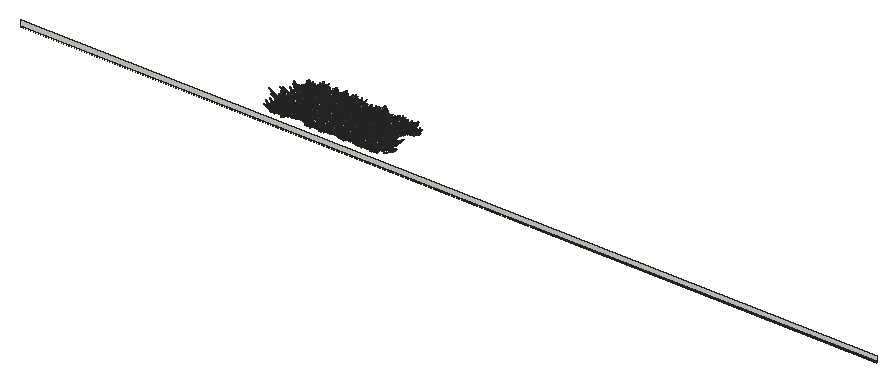
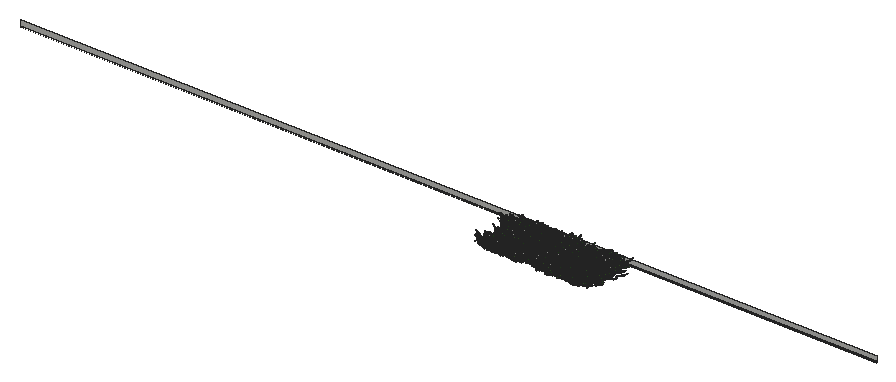
# SketchUp Ruby script. Lengths in inches.
U = 1.inch
M = Sketchup.active_model
def pt(a) = Geom::Point3d.new(a.map { |v| v * U })
def face(e, loops, mat)
  f = e.add_face(loops[0].map { |a| pt(a) })
  loops[1..].each { |l| e.add_face(l.map { |a| pt(a) }).erase! }
  f.material = f.back_material = mat if mat
  f
end
# faces: each face lists its corners as indices into pts; further lists are holes
def faces(e, pts, list, mat = nil) = list.each { |f| face(e, (f[0].is_a?(Array) ? f : [f]).map { |l| l.map { |i| pts[i] } }, mat) }
# xy, xz, yz: faces in a plane at the given z, y or x. An outline is a flat list of corners, or four numbers for a rectangle; further outlines are holes
def ring(l) = l.size == 4 ? [[l[0], l[1]], [l[2], l[1]], [l[2], l[3]], [l[0], l[3]]] : l.each_slice(2).to_a
def flat(e, list, mat, &to3) = list.each { |f| face(e, (f[0].is_a?(Array) ? f : [f]).map { |l| ring(l).map { |u, v| to3.(u, v) } }, mat) }
def xy(e, z, list, mat = nil) = flat(e, list, mat) { |x, y| [x, y, z] }
def xz(e, y, list, mat = nil) = flat(e, list, mat) { |x, z| [x, y, z] }
def yz(e, x, list, mat = nil) = flat(e, list, mat) { |y, z| [x, y, z] }
def lines(e, pts, list) = list.each { |a, b| e.add_line(pt(pts[a]), pt(pts[b])) }
# prism: a flat outline (further loops are holes) pulled along v
def prism(e, loops, v, mat = nil)
  f = face(e, loops, mat); d = Geom::Vector3d.new(v.map { |x| x * U })
  f.pushpull(f.normal.samedirection?(d) ? d.length : -d.length)
end
def box(e, o, s, mat = nil) = prism(e, [[o, [o[0] + s[0], o[1], o[2]], [o[0] + s[0], o[1] + s[1], o[2]], [o[0], o[1] + s[1], o[2]]]], [0, 0, s[2]], mat)
def at(x, y, z, deg = 0) = Geom::Transformation.translation(pt([x, y, z])) * Geom::Transformation.rotation(ORIGIN, Z_AXIS, deg.degrees)
def axes(o, x, y, z) = Geom::Transformation.new([*x, 0, *y, 0, *z, 0, *pt(o).to_a, 1])
def part(name) = M.definitions.add(name)
# library, detail: a bought-in or finely detailed component or shape, given as its bounding box
def library(name, o, s) = part(name).tap { |d| box(d.entities, o, s) }
def detail(e, o, s) = box(e.add_group.entities, o, s)
def put(e, d, t, mat = nil) = e.add_instance(d, t).tap { |i| i.material = mat if mat }
def group(e, t, mat = nil) = e.add_group.tap { |g| g.transformation = t; g.material = mat if mat }.entities
root = M.entities
M.materials.add("Material82").color = [68, 110, 58]
M.materials.add("Material83").color = [48, 90, 38]
M.materials.add("Material84").color = [68, 110, 48]
M.materials.add("Material85").color = [48, 90, 48]
M.materials.add("Material86").color = [58, 110, 58]
M.materials.add("Material87").color = [58, 90, 38]
M.materials.add("Material88").color = [68, 100, 58]
M.materials.add("Material89").color = [48, 100, 38]
c1 = part("grass00")
p = [[-0.6875,0.15,0],[-0.56,0.08,5.52],[-0.04,0.03,2.76],[0.48,-0.02,0],[0.35,-0.02,5.52],[-0.1,-0.14,5.52],
  [-0.12,0.65,8.37],[-0.42,0.65,8.37]]
faces(c1.entities,p,[[0,1,2,3],[3,2,4],[1,5,2],[5,4,2],[1,6,5],[4,5,6],[7,6,1]])
c2 = part("Group16\#1")
put(c2.entities,c1,axes([1.44,-0.61,-0.01],[0.05352,0.12609,0],[-0.10704,0.04543,0.07239],[0.06664,-0.02828,0.11628]),"Material85")
put(c2.entities,c1,axes([0.76,-0.15,-0.01],[0.04676,0.24062,0],[-0.23162,0.04501,0.06642],[0.0652,-0.01267,0.23595]),"Material82")
put(c2.entities,c1,axes([0.79,0.01,-0.01],[-0.00606,0.34651,0],[-0.34381,-0.00602,0.0432],[0.04319,0.00076,0.34386]))
put(c2.entities,c1,axes([1,0.23,-0.01],[-0.07192,0.31144,0],[-0.28722,-0.06632,0.1236],[0.12043,0.02781,0.29478]),"Material84")
put(c2.entities,c1,axes([1.66,0.77,-0.01],[-0.13828,0.29651,0],[-0.21551,-0.1005,0.22471],[0.20365,0.09498,0.23779]),"Material89")
put(c2.entities,c1,axes([0.6875,0.52,-0.01],[-0.18126,0.24051,0],[-0.22746,-0.17142,0.09788],[0.07817,0.05891,0.28481]),"Material84")
put(c2.entities,c1,axes([0.68,0.78,-0.01],[-0.215,0.18688,0],[-0.12385,-0.14248,0.21334],[0.13995,0.16101,0.18878]),"Material82")
put(c2.entities,c1,axes([0.56,1,-0.01],[-0.13756,0.07624,0],[-0.06159,-0.11112,0.0927],[0.04494,0.08108,0.12705]),"Material84")
put(c2.entities,c1,axes([0.2,0.64,-0.01],[-0.23729,0.07254,0],[-0.05711,-0.18681,0.153],[0.04473,0.14632,0.19535]),"Material89")
put(c2.entities,c1,axes([0.0625,0.72,-0.01],[-0.28874,0.02525,0],[-0.02179,-0.24916,0.14647],[0.01276,0.14591,0.25012]),"Material82")
put(c2.entities,c1,axes([-0.08,0.62,-0.01],[-0.34089,-0.04187,0],[0.03255,-0.26504,0.216],[-0.02633,0.21439,0.26703]),"Material89")
put(c2.entities,c1,axes([-0.34,0.98,-0.01],[-0.14314,-0.0493,0],[0.04397,-0.12769,0.06843],[-0.02228,0.0647,0.13505]),"Material89")
put(c2.entities,c1,axes([-0.87,1.45,-0.01],[-0.23488,-0.14114,0],[0.13761,-0.22901,0.06087],[-0.03135,0.05217,0.26717]))
put(c2.entities,c1,axes([-0.72,0.77,-0.01],[-0.14208,-0.13251,0],[0.07209,-0.0773,0.16301],[-0.11118,0.11922,0.1057]),"Material89")
put(c2.entities,c1,axes([-0.62,0.43,-0.01],[-0.14845,-0.21203,0],[0.18654,-0.13061,0.12304],[-0.10079,0.07057,0.22772]),"Material82")
put(c2.entities,c1,axes([-0.68,0.29,-0.01],[-0.13639,-0.32136,0],[0.31723,-0.13464,0.05579],[-0.05136,0.0218,0.34462]),"Material83")
put(c2.entities,c1,axes([-0.64,0.125,-0.01],[-0.0458,-0.23569,0],[0.22124,-0.043,0.08276],[-0.08124,0.01579,0.22538]),"Material86")
put(c2.entities,c1,axes([-1.6,-0.03,-0.01],[0.00576,-0.32897,0],[0.27526,0.00482,0.18018],[-0.18015,-0.00315,0.2753]),"Material84")
put(c2.entities,c1,axes([-1.36,-0.31,-0.01],[0.05718,-0.24765,0],[0.18172,0.04196,0.17267],[-0.16825,-0.03885,0.1865]),"Material89")
put(c2.entities,c1,axes([-1.54,-0.72,-0.01],[0.06537,-0.14017,0],[0.13555,0.06321,0.03939],[-0.0357,-0.01665,0.14956]))
put(c2.entities,c1,axes([-1.19,-0.9,-0.01],[0.09597,-0.12735,0],[0.11214,0.08451,0.07557],[-0.06035,-0.04548,0.14042]),"Material88")
put(c2.entities,c1,axes([-0.47,-0.54,-0.01],[0.11588,-0.10072,0],[0.0618,0.0711,0.12124],[-0.07953,-0.0915,0.0942]))
put(c2.entities,c1,axes([-0.47,-0.84,-0.01],[0.11927,-0.0661,0],[0.06603,0.11913,0.00646],[-0.00313,-0.00565,0.13621]),"Material84")
put(c2.entities,c1,axes([-0.38,-1.24,-0.01],[0.28037,-0.08571,0],[0.0618,0.20215,0.20315],[-0.05939,-0.19428,0.21139]),"Material88")
put(c2.entities,c1,axes([-0.06,-0.66,-0.01],[0.22719,-0.01987,0],[0.01247,0.14255,0.17758],[-0.01547,-0.17691,0.1431]),"Material87")
put(c2.entities,c1,axes([0.11,-0.89,-0.01],[0.14882,0.01828,0],[-0.01058,0.08611,0.12229],[0.01491,-0.12138,0.08676]),"Material85")
put(c2.entities,c1,axes([0.25,-0.72,-0.01],[0.20481,0.07053,0],[-0.06206,0.18022,0.10291],[0.03351,-0.0973,0.1906]),"Material85")
put(c2.entities,c1,axes([0.85,-1.42,-0.01],[0.16481,0.09904,0],[-0.09472,0.15762,0.05616],[0.02893,-0.04814,0.18389]),"Material84")
put(c2.entities,c1,axes([1.01,-1.09,-0.01],[0.21858,0.20385,0],[-0.17495,0.1876,0.15339],[0.10462,-0.11218,0.25652]),"Material89")
put(c2.entities,c1,axes([1.01,-0.71,-0.01],[0.08733,0.12473,0],[-0.06445,0.04512,0.13037],[0.1068,-0.07477,0.07867]),"Material85")
c3 = part("Group15\#1")
put(c3.entities,c2,at(0,0,0))
c4 = part("3darcstudiotree_grass00\#1")
put(c4.entities,c3,at(0,0,0))
xz(root,273.41,[[1534.73,-38.1875,2096.97,-37.86],[1534.73,-37.24,2096.97,-34.17]])
put(root,c4,axes([1753.47,281.1875,-34.17],[2.17079,-1.3067,0],[3.53732,0.91396,-0.04807],[0.21538,0.05565,1.69791]))
put(root,c4,axes([1759.32,281.2,-34.17],[4.07054,-0.47424,0],[1.26442,1.68794,-0.05518],[0.08285,0.1106,1.77288]))
put(root,c4,axes([1699.04,281.26,-34.17],[0.55958,-1.81201,0],[3.80263,0.18264,-0.0324],[0.16574,0.00796,1.47946]))
put(root,c4,axes([1722.34,281.33,-34.17],[1.12764,-1.73077,0],[4.18377,0.42395,-0.01129],[0.06303,0.00639,1.86628]))
put(root,c4,axes([1743.74,281.47,-34.17],[1.22394,-1.54587,0],[4.34445,0.53497,-0.04262],[0.21661,0.02667,1.81655]))
put(root,c4,axes([1732.14,281.62,-34.17],[-3.03372,-1.40875,0],[3.08967,-1.03482,-0.05304],[0.26,-0.08708,1.95407]))
put(root,c4,axes([1727.11,282.65,-34.17],[1.40551,-1.64885,0],[4.26228,0.56508,-0.02131],[0.10181,0.0135,1.69918]))
put(root,c4,axes([1731.34,282.95,-34.17],[1.31732,-1.5277,0],[3.94533,0.52911,-0.01889],[0.1126,0.0151,1.96679]))
put(root,c4,axes([1754.46,283.05,-34.17],[1.63405,-1.64828,0],[3.24927,0.50099,-0.00888],[0.05923,0.00913,1.87213]))
put(root,c4,axes([1701,282.59,-34.17],[-3.98203,-0.87024,0],[2.1917,-1.55976,-0.02403],[0.066,-0.04697,1.92026]))
put(root,c4,axes([1748.21,282.77,-34.17],[-3.61082,-0.39433,0],[1.20081,-1.71014,-0.02644],[0.03989,-0.05681,1.9068]))
put(root,c4,axes([1710.51,282.87,-34.17],[-3.87962,-0.67736,0],[1.4284,-1.27243,-0.0129],[0.02606,-0.02321,1.31952]))
put(root,c4,axes([1745.46,283.12,-34.17],[3.46015,0.38109,0],[-0.88814,1.25417,-0.03829],[-0.05842,0.0825,1.40372]))
put(root,c4,axes([1740.78,282.8,-34.17],[-3.41936,-0.32293,0],[0.80872,-1.33182,-0.00326],[0.00565,-0.00931,1.93944]))
put(root,c4,axes([1723.11,283.16,-34.17],[3.02481,0.98705,0],[-2.84435,1.35567,-0.00662],[-0.02068,0.00986,1.63949]))
put(root,c4,axes([1718.68,283.8,-34.17],[0.88446,1.28365,0],[-3.4154,0.366,-0.02204],[-0.14997,0.01607,1.87051]))
put(root,c4,axes([1705.0625,283.9,-34.17],[-0.33098,1.70392,0],[-3.92143,-0.11847,-0.03234],[-0.20787,-0.00628,1.90052]))
put(root,c4,axes([1705.14,284.73,-34.17],[4.23456,-0.44217,0],[1.03247,1.53783,-0.03329],[0.03822,0.05692,1.35616]))
put(root,c4,axes([1753.52,284.58,-34.17],[-1.01765,1.47435,0],[-4.56253,-0.4898,-0.0223],[-0.09653,-0.01036,1.58974]))
put(root,c4,axes([1712.44,284.81,-34.17],[0.47172,1.49628,0],[-3.52699,0.17294,-0.00588],[-0.02991,0.00147,1.36568]))
put(root,c4,axes([1760.9,285.43,-34.17],[0.9992,-1.70874,0],[3.78612,0.34433,-0.00305],[0.01806,0.00164,1.76865]))
put(root,c4,axes([1735.08,285.14,-34.17],[-3.90096,-0.14279,0],[0.42836,-1.82008,-0.06502],[0.0247,-0.10495,1.42798]))
put(root,c4,axes([1749.08,285.56,-34.17],[4.57837,0.42186,0],[-0.79113,1.33536,-0.04207],[-0.04884,0.08244,1.32997]))
put(root,c4,axes([1717.02,285.52,-34.17],[1.5336,1.30723,0],[-4.13356,0.75421,-0.03574],[-0.18177,0.03317,1.91331]))
put(root,c4,axes([1722.26,286,-34.17],[3.57543,-0.38769,0],[0.94849,1.36047,-0.03828],[0.05948,0.08532,1.57185]))
put(root,c4,axes([1743.97,286.02,-34.17],[3.20776,-0.47754,0],[1.28857,1.34619,-0.04981],[0.10847,0.11332,1.68613]))
put(root,c4,axes([1726.58,285.74,-34.17],[0.98392,1.60393,0],[-4.31274,0.41147,-0.01063],[-0.04621,0.00441,1.48723]))
put(root,c4,axes([1698.96,286.05,-34.17],[-2.94402,-0.61655,0],[1.96985,-1.46292,-0.05452],[0.11404,-0.08469,1.404]))
put(root,c4,axes([1761.52,286.76,-34.17],[0.83554,-1.66698,0],[4.46376,0.34798,-0.04547],[0.22573,0.0176,1.72572]))
put(root,c4,axes([1739.54,286.08,-34.17],[-4.29885,0.51765,0],[-1.3445,-1.73657,-0.03433],[-0.03931,-0.05078,1.35329]))
put(root,c4,axes([1745.2,286.72,-34.17],[-0.83396,-1.47678,0],[3.24144,-0.28469,-0.00779],[0.04244,-0.00373,1.38852]))
put(root,c4,axes([1749.99,287,-34.17],[0.8669,-1.63737,0],[4.38165,0.36081,-0.01659],[0.07514,0.00619,1.55232]))
put(root,c4,axes([1734.67,286.9,-34.17],[2.831,1.13552,0],[-3.26481,1.26594,-0.00938],[-0.03813,0.01479,1.95578]))
put(root,c4,axes([1727.38,286.87,-34.17],[2.31946,1.24356,0],[-3.54601,1.02866,-0.02079],[-0.06877,0.01995,1.35493]))
put(root,c4,axes([1716.98,287.19,-34.17],[3.58882,-0.43849,0],[1.01017,1.28588,-0.04073],[0.06773,0.08621,1.43775]))
put(root,c4,axes([1710.05,287.42,-34.17],[3.87508,-0.19158,0],[0.55593,1.74888,-0.03701],[0.02742,0.08626,1.99511]))
put(root,c4,axes([1755.1,286.81,-34.17],[-1.66334,1.46333,0],[-4.128,-0.72978,-0.00369],[-0.01567,-0.00277,1.57624]))
put(root,c4,axes([1701.35,287.47,-34.17],[-2.23453,-0.97852,0],[2.77364,-0.9851,-0.04825],[0.23755,-0.08437,1.85346]))
put(root,c4,axes([1737.07,288.01,-34.17],[0.13943,1.51336,0],[-3.52829,0.05056,-0.04285],[-0.2957,0.00424,1.82733]))
put(root,c4,axes([1722.85,287.92,-34.17],[-2.1552,1.3099,0],[-3.57978,-0.91604,-0.05659],[-0.20761,-0.05313,1.39892]))
put(root,c4,axes([1706.03,288.18,-34.17],[-3.02099,1.21639,0],[-3.37871,-1.30508,-0.0181],[-0.07062,-0.02728,1.93624]))
put(root,c4,axes([1712.21,288.95,-34.17],[4.11072,0.52115,0],[-1.12592,1.38127,-0.00634],[-0.01225,0.01503,1.74238]))
put(root,c4,axes([1699.97,289.22,-34.17],[1.39356,-1.72752,0],[4.38256,0.54985,-0.00448],[0.02218,0.00278,1.79011]))
put(root,c4,axes([1759.64,289.61,-34.17],[-0.53843,-1.61653,0],[3.48383,-0.18047,-0.04534],[0.27707,-0.01435,1.62314]))
put(root,c4,axes([1754.86,289.17,-34.17],[-1.88196,1.3957,0],[-3.10758,-0.65171,-0.04799],[-0.32006,-0.06712,1.99284]))
put(root,c4,axes([1704.65,289.95,-34.17],[0.57397,-1.69302,0],[4.41794,0.23295,-0.0102],[0.05353,0.00282,1.76846]))
put(root,c4,axes([1738.95,289.83,-34.17],[-0.52019,-1.47295,0],[3.61124,-0.19836,-0.01078],[0.07028,-0.00386,1.79898]))
put(root,c4,axes([1742.48,289.66,-34.17],[-0.97814,1.51943,0],[-3.80237,-0.3807,-0.01715],[-0.08253,-0.00826,1.46021]))
put(root,c4,axes([1724.19,289.77,-34.17],[0.84595,1.74988,0],[-3.45616,0.25986,-0.03349],[-0.2005,0.01508,1.60736]))
put(root,c4,axes([1715.28,290,-34.17],[-3.51608,0.58555,0],[-1.76508,-1.64843,-0.01449],[-0.02729,-0.02549,1.64714]))
put(root,c4,axes([1751.16,290.39,-34.17],[2.67266,1.37649,0],[-3.28703,0.99263,-0.02004],[-0.06999,0.02114,1.3651]))
put(root,c4,axes([1725.6875,290.53,-34.17],[-2.74028,-0.81988,0],[2.08475,-1.08371,-0.01586],[0.05642,-0.02933,1.52204]))
put(root,c4,axes([1731.9375,290.22,-34.17],[-2.48253,1.23787,0],[-2.67891,-0.83558,-0.01059],[-0.04346,-0.01356,1.33934]))
put(root,c4,axes([1728.22,291.375,-34.17],[-3.00354,-1.31894,0],[3.37135,-1.19405,-0.05274],[0.22952,-0.08129,1.98669]))
put(root,c4,axes([1735.15,291.86,-34.17],[1.37504,-1.64012,0],[4.21946,0.55019,-0.04027],[0.19656,0.02563,1.71232]))
put(root,c4,axes([1751.53,292.11,-34.17],[2.76982,-1.52047,0],[2.85461,0.80878,-0.0087],[0.04308,0.01221,1.60603]))
put(root,c4,axes([1711.15,292.1875,-34.17],[2.88399,-0.92183,0],[2.75264,1.33938,-0.02341],[0.07157,0.03482,1.59067]))
put(root,c4,axes([1722.84,291.59,-34.17],[-4.47684,0.54828,0],[-1.1065,-1.40519,-0.03919],[-0.07055,-0.08959,1.69748]))
put(root,c4,axes([1753.65,291.6,-34.17],[-4.11453,0.51388,0],[-1.13165,-1.40923,-0.01419],[-0.02668,-0.03323,1.75006]))
put(root,c4,axes([1737.4,291.6875,-34.17],[-4.23608,0.30685,0],[-0.85226,-1.82987,-0.05609],[-0.05564,-0.11947,1.94158]))
put(root,c4,axes([1745.36,291.95,-34.17],[2.07706,1.01263,0],[-2.63538,0.84072,-0.02717],[-0.1514,0.0483,1.82093]))
put(root,c4,axes([1759.7,291.98,-34.17],[-3.63945,-0.58666,0],[1.30533,-1.25945,-0.04864],[0.1019,-0.09832,1.4319]))
put(root,c4,axes([1706.06,292.07,-34.17],[-4.25916,-0.67423,0],[1.26133,-1.23925,-0.04034],[0.09396,-0.09232,1.58691]))
put(root,c4,axes([1698.41,291.66,-34.17],[-3.70599,0.79197,0],[-2.20745,-1.60656,-0.0133],[-0.03552,-0.02585,1.94738]))
put(root,c4,axes([1714.98,292.51,-34.17],[-4.16919,-0.21002,0],[0.49933,-1.5417,-0.0157],[0.01299,-0.04011,1.92971]))
put(root,c4,axes([1699.76,293.28,-34.17],[-0.43315,-1.7077,0],[3.80872,-0.15025,-0.05423],[0.31945,-0.0126,1.69842]))
put(root,c4,axes([1722.02,293.84,-34.17],[1.31559,-1.26739,0],[3.71813,0.60026,-0.00546],[0.02236,0.00361,1.33158]))
put(root,c4,axes([1733.34,293.35,-34.17],[0.02685,1.39613,0],[-4.67009,0.01397,-0.03677],[-0.14547,0.00044,1.38481]))
put(root,c4,axes([1729.65,293.98,-34.17],[2.75881,-1.06303,0],[3.05708,1.23394,-0.03867],[0.14354,0.05794,1.7417]))
put(root,c4,axes([1711.7,293.77,-34.17],[-1.10259,-1.32087,0],[4.19794,-0.54501,-0.05688],[0.29749,-0.03862,1.82396]))
put(root,c4,axes([1757.14,294.25,-34.17],[0.84647,-1.73268,0],[3.98325,0.30265,-0.00212],[0.01137,0.00086,1.6588]))
put(root,c4,axes([1750.33,293.55,-34.17],[-2.78854,1.36928,0],[-2.88748,-0.91457,-0.04358],[-0.20411,-0.06465,1.66757]))
put(root,c4,axes([1737.88,294.65,-34.17],[3.75686,0.07381,0],[-0.21994,1.74119,-0.00527],[-0.00126,0.00998,1.59512]))
put(root,c4,axes([1703.72,294.69,-34.17],[2.35188,-1.38482,0],[3.12769,0.82614,-0.05113],[0.23612,0.06237,1.56833]))
put(root,c4,axes([1743.79,294.06,-34.17],[-2.45653,1.59128,0],[-3.13753,-0.75331,-0.03488],[-0.14833,-0.03561,1.37068]))
put(root,c4,axes([1715.22,294.87,-34.17],[0.70204,1.43301,0],[-3.58325,0.27302,-0.03785],[-0.19362,0.01475,1.42505]))
put(root,c4,axes([1751.76,296.27,-34.17],[3.07151,-0.57195,0],[1.60637,1.34169,-0.03456],[0.08725,0.07287,1.66747]))
put(root,c4,axes([1745.32,296.33,-34.17],[0.41064,-1.32496,0],[4.30887,0.2077,-0.02785],[0.12721,0.00613,1.49696]))
put(root,c4,axes([1715.5625,296.54,-34.17],[3.86131,0.54377,0],[-1.4335,1.58316,-0.00059],[-0.00108,0.0012,1.74794]))
put(root,c4,axes([1712.33,296.25,-34.17],[-3.05685,-0.82947,0],[2.14696,-1.23058,-0.02104],[0.07287,-0.04177,1.73448]))
put(root,c4,axes([1726.47,296.72,-34.17],[2.41246,-1.41032,0],[3.04441,0.80995,-0.04469],[0.24595,0.06543,1.8275]))
put(root,c4,axes([1733.72,296.81,-34.17],[3.60532,-0.46019,0],[1.33734,1.62954,-0.01611],[0.02411,0.02937,1.58139]))
put(root,c4,axes([1724.16,296.47,-34.17],[3.77018,0.78532,0],[-1.755,1.3104,-0.05015],[-0.15166,0.11324,1.82381]))
put(root,c4,axes([1739.39,296.2,-34.17],[-0.64515,1.28427,0],[-4.09885,-0.32024,-0.03573],[-0.18751,-0.01465,1.67549]))
put(root,c4,axes([1703.53,296.27,-34.17],[-3.1964,-0.45712,0],[1.21547,-1.32188,-0.00444],[0.00788,-0.00857,1.39182]))
put(root,c4,axes([1755.83,296.61,-34.17],[-3.33624,1.28886,0],[-2.34327,-0.94338,-0.00183],[-0.00717,-0.00289,1.40539]))
put(root,c4,axes([1699.84,296.92,-34.17],[-3.35036,0.87409,0],[-2.07562,-1.23735,-0.03289],[-0.10016,-0.05971,1.55622]))
put(root,c4,axes([1710.98,298,-34.17],[2.33049,-1.15129,0],[2.65609,0.83622,-0.01018],[0.04728,0.01488,1.51436]))
put(root,c4,axes([1733.08,297.63,-34.17],[2.78328,1.41625,0],[-3.60575,1.10211,-0.03267],[-0.14651,0.04478,1.93988]))
put(root,c4,axes([1703.79,297.84,-34.17],[2.67683,1.25305,0],[-2.64635,0.87925,-0.04423],[-0.18001,0.05981,1.38013]))
put(root,c4,axes([1699.87,298.33,-34.17],[4.04553,0.2871,0],[-0.83462,1.82911,-0.01866],[-0.01606,0.0352,1.717]))
put(root,c4,axes([1749.2,297.9,-34.17],[1.39252,1.41751,0],[-3.18673,0.48689,-0.02409],[-0.14094,0.02153,1.60735]))
put(root,c4,axes([1720.25,298.12,-34.17],[-4.2844,-0.03587,0],[0.08793,-1.63328,-0.04949],[0.00646,-0.12004,1.9102]))
put(root,c4,axes([1717.21,298.36,-34.17],[-4.02551,-0.90949,0],[2.09135,-1.43967,-0.04075],[0.0999,-0.06877,1.55523]))
put(root,c4,axes([1729.04,298.9,-34.17],[4.10034,-0.52862,0],[1.2552,1.51427,-0.04269],[0.08479,0.10229,1.93529]))
put(root,c4,axes([1743.35,298.92,-34.17],[3.38301,-0.17676,0],[0.47183,1.40447,-0.04905],[0.03546,0.10554,1.48186]))
put(root,c4,axes([1739.29,298.85,-34.17],[2.80686,0.98493,0],[-2.35719,1.04478,-0.00943],[-0.03285,0.01456,1.39243]))
put(root,c4,axes([1755.9,298.96,-34.17],[-1.98727,-1.58329,0],[3.14557,-0.61406,-0.01272],[0.05955,-0.01163,1.37453]))
put(root,c4,axes([1714.74,299.92,-34.17],[0.60335,-1.83981,0],[4.64218,0.23677,-0.05291],[0.19949,0.01017,1.33374]))
put(root,c4,axes([1731.84,299.86,-34.17],[-3.10894,1.29688,0],[-2.64938,-0.9878,-0.02847],[-0.10631,-0.03964,1.40417]))
put(root,c4,axes([1711.61,300.61,-34.17],[2.49775,-0.87161,0],[2.87959,1.28342,-0.04815],[0.19249,0.08579,1.9649]))
put(root,c4,axes([1750.84,301.15,-34.17],[3.6923,-0.26906,0],[0.83055,1.77269,-0.01263],[0.0116,0.02476,1.73191]))
put(root,c4,axes([1756.54,300.86,-34.17],[-2.8282,-0.92386,0],[2.41261,-1.14869,-0.01497],[0.06145,-0.02926,1.82381]))
put(root,c4,axes([1742.49,301.11,-34.17],[-1.60359,-1.29455,0],[3.30864,-0.63743,-0.0349],[0.20941,-0.04034,1.84302]))
put(root,c4,axes([1721.17,301.23,-34.17],[3.05854,0.58726,0],[-2.04234,1.65433,-0.05845],[-0.11264,0.09124,1.53958]))
put(root,c4,axes([1704.9375,301.0625,-34.17],[-3.29694,-0.59268,0],[1.38855,-1.20133,-0.0331],[0.08455,-0.07315,1.54531]))
put(root,c4,axes([1737.66,301.43,-34.17],[-3.83901,-0.76558,0],[1.48905,-1.16132,-0.0255],[0.09039,-0.0705,1.94297]))
put(root,c4,axes([1725.875,301.18,-34.17],[-1.85089,1.19146,0],[-2.90652,-0.70224,-0.01687],[-0.07661,-0.01851,1.36079]))
put(root,c4,axes([1737.5625,302.28,-34.17],[3.52935,-0.50726,0],[1.49485,1.61761,-0.06136],[0.11602,0.12555,1.80687]))
put(root,c4,axes([1700.57,302.19,-34.17],[-2.79186,-1.03231,0],[2.26214,-0.95152,-0.04465],[0.21173,-0.08906,1.71883]))
put(root,c4,axes([1723.93,302.4375,-34.17],[4.31211,0.22009,0],[-0.60247,1.83583,-0.04718],[-0.02535,0.07723,1.4726]))
put(root,c4,axes([1760.02,302.75,-34.17],[0.02414,-1.32822,0],[3.48081,0.00984,-0.01704],[0.11733,0.00033,1.79616]))
put(root,c4,axes([1726.66,303.14,-34.17],[1.88589,-1.60822,0],[4.27567,0.77981,-0.01],[0.0511,0.00932,1.98774]))
put(root,c4,axes([1734.125,302.54,-34.17],[-0.58657,1.2788,0],[-3.43074,-0.24475,-0.01415],[-0.07642,-0.00545,1.43376]))
put(root,c4,axes([1750.16,302.91,-34.17],[4.10063,0.83805,0],[-2.12312,1.61572,-0.0509],[-0.10915,0.08307,1.61215]))
put(root,c4,axes([1706.74,303.24,-34.17],[1.13928,-1.32787,0],[4.00016,0.53378,-0.02846],[0.11467,0.0153,1.34635]))
put(root,c4,axes([1710.16,303.28,-34.17],[4.20126,0.39077,0],[-0.91213,1.52518,-0.02883],[-0.04091,0.06841,1.84132]))
put(root,c4,axes([1744.42,302.92,-34.17],[-2.19345,1.65823,0],[-4.03021,-0.82913,-0.04188],[-0.20563,-0.0423,1.88687]))
put(root,c4,axes([1756.52,303.36,-34.17],[2.38559,0.94842,0],[-2.99836,1.17298,-0.03885],[-0.13848,0.05417,1.58937]))
put(root,c4,axes([1714.95,303.55,-34.17],[-1.58706,-1.22315,0],[3.88697,-0.78439,-0.02541],[0.09132,-0.01843,1.32108]))
put(root,c4,axes([1720.87,304.22,-34.17],[2.23016,-1.08828,0],[2.80047,0.89256,-0.01488],[0.0583,0.01858,1.35946]))
put(root,c4,axes([1750.56,304.34,-34.17],[3.39127,-1.14999,0],[2.14538,0.98397,-0.0226],[0.09906,0.04544,1.65792]))
put(root,c4,axes([1713.09,304.7,-34.17],[3.24027,-0.98547,0],[2.31887,1.18584,-0.00737],[0.02262,0.01157,1.42978]))
put(root,c4,axes([1737.35,304.72,-34.17],[-0.94888,-1.39552,0],[4.53946,-0.48005,-0.04199],[0.20499,-0.02168,1.7807]))
put(root,c4,axes([1753.63,305.09,-34.17],[2.51974,-1.17528,0],[3.05999,1.02034,-0.03628],[0.13748,0.04584,1.49031]))
put(root,c4,axes([1707.21,305.03,-34.17],[1.43898,-1.34623,0],[3.17438,0.52772,-0.03331],[0.18037,0.02999,1.51731]))
put(root,c4,axes([1744.34,304.33,-34.17],[-4.29208,0.36507,0],[-0.8528,-1.5594,-0.00845],[-0.00798,-0.0146,1.35873]))
put(root,c4,axes([1699.08,304.67,-34.17],[-3.56566,-0.8896,0],[2.32838,-1.45148,-0.01513],[0.04457,-0.02778,1.79885]))
put(root,c4,axes([1727.59,305.03,-34.17],[2.9165,0.98147,0],[-2.52132,1.16527,-0.03219],[-0.13562,0.06268,1.88986]))
put(root,c4,axes([1714.6875,305.125,-34.17],[2.05839,1.31648,0],[-3.03228,0.73739,-0.00763],[-0.03853,0.00937,1.58363]))
put(root,c4,axes([1760.09,305.53,-34.17],[-2.38248,1.06709,0],[-3.21771,-1.11734,-0.02335],[-0.09118,-0.03166,1.67208]))
put(root,c4,axes([1733.38,305.62,-34.17],[-3.50072,1.23157,0],[-2.52643,-1.11691,-0.04505],[-0.14682,-0.06491,1.39266]))
put(root,c4,axes([1760.76,306.61,-34.17],[2.50615,-1.32245,0],[2.94011,0.86656,-0.03861],[0.1979,0.05833,1.76068]))
put(root,c4,axes([1718.62,306.58,-34.17],[1.26993,-1.49927,0],[3.12751,0.41201,-0.03453],[0.23339,0.03075,1.76116]))
put(root,c4,axes([1707.37,306.36,-34.17],[1.96702,1.06284,0],[-3.17968,0.91525,-0.05552],[-0.21201,0.06102,1.39481]))
put(root,c4,axes([1755.61,306.66,-34.17],[-1.89774,-1.54823,0],[3.70179,-0.70571,-0.04214],[0.19197,-0.0366,1.55921]))
put(root,c4,axes([1700.02,306.42,-34.17],[-3.34111,0.18713,0],[-0.56421,-1.56678,-0.00819],[-0.00515,-0.01431,1.3463]))
put(root,c4,axes([1749.63,306.93,-34.17],[3.59081,0.56064,0],[-1.39714,1.39174,-0.03237],[-0.06842,0.06816,1.63378]))
put(root,c4,axes([1723.93,307.3,-34.17],[2.80865,-0.79423,0],[2.35611,1.29587,-0.04704],[0.15431,0.08487,1.70604]))
put(root,c4,axes([1740.03,306.65,-34.17],[-0.90085,1.67926,0],[-4.44806,-0.37112,-0.05558],[-0.25392,-0.02119,1.59125]))
put(root,c4,axes([1711.125,307.52,-34.17],[1.64847,-1.35078,0],[4.23243,0.80334,-0.06017],[0.26789,0.05085,1.73941]))
put(root,c4,axes([1734.58,307.15,-34.17],[-4.10859,0.05118,0],[-0.12582,-1.57107,-0.03959],[-0.00691,-0.08629,1.65212]))
put(root,c4,axes([1744.01,307.24,-34.17],[-2.91157,1.30067,0],[-2.86972,-0.9991,-0.01581],[-0.05499,-0.01914,1.33135]))
put(root,c4,axes([1729.27,307.47,-34.17],[-0.60337,1.5081,0],[-3.83662,-0.23874,-0.0149],[-0.0971,-0.00604,1.9212]))
put(root,c4,axes([1760.42,308.59,-34.17],[-1.25473,-1.49042,0],[3.70912,-0.48565,-0.03393],[0.14523,-0.01902,1.3212]))
put(root,c4,axes([1710.49,308.67,-34.17],[-4.49573,0.21611,0],[-0.44378,-1.43584,-0.03065],[-0.02667,-0.0863,1.97713]))
put(root,c4,axes([1749.8,309.21,-34.17],[-2.33047,-0.97071,0],[3.43186,-1.28143,-0.06171],[0.20646,-0.07709,1.63202]))
put(root,c4,axes([1721.71,309.54,-34.17],[4.02075,-0.11832,0],[0.27482,1.45248,-0.02534],[0.01078,0.05696,1.58232]))
put(root,c4,axes([1740.3,309.14,-34.17],[1.7612,1.59038,0],[-3.40002,0.5856,-0.01938],[-0.1015,0.01748,1.58937]))
put(root,c4,axes([1704.07,309.6875,-34.17],[1.1756,-1.47793,0],[3.44657,0.42639,-0.02865],[0.17647,0.02183,1.74795]))
put(root,c4,axes([1756.4,309.15,-34.17],[-3.12054,0.56833,0],[-1.82234,-1.55622,-0.05064],[-0.09583,-0.08183,1.47033]))
put(root,c4,axes([1717.27,310.05,-34.17],[2.53276,-1.11904,0],[3.44801,1.21375,-0.02458],[0.09462,0.03331,1.78746]))
put(root,c4,axes([1725.7,310.15,-34.17],[3.19182,-1.13301,0],[2.43556,1.06713,-0.02235],[0.10598,0.04644,1.93391]))
put(root,c4,axes([1701.55,309.8,-34.17],[2.22198,1.23467,0],[-3.2898,0.92081,-0.0048],[-0.02055,0.00575,1.58899]))
